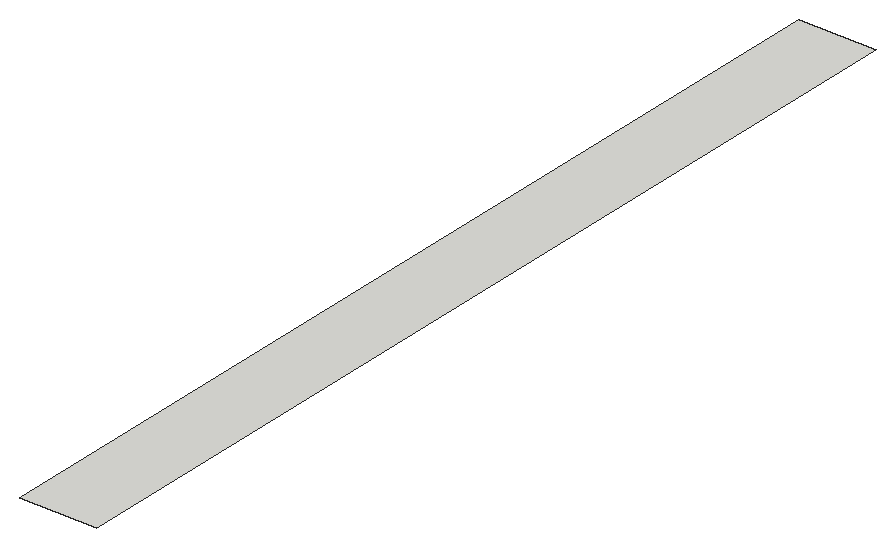
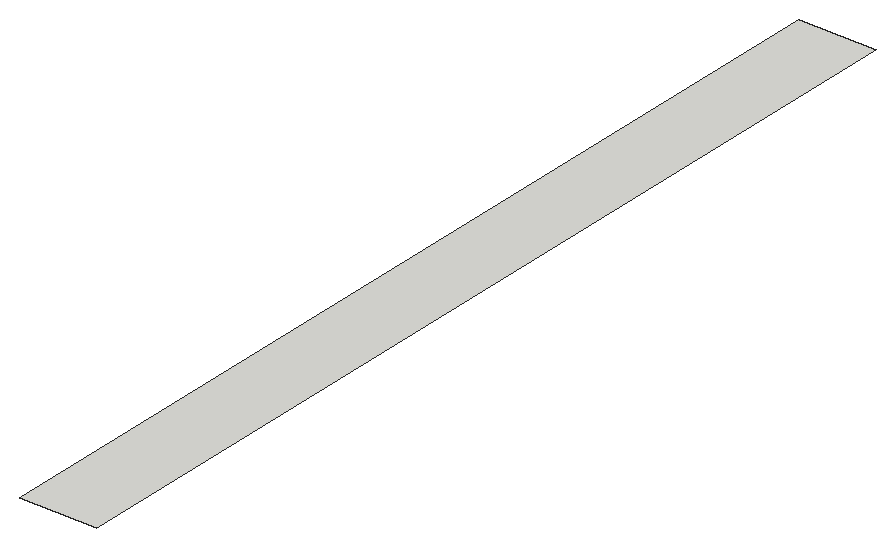
# SketchUp Ruby script. Lengths in inches.
U = 1.inch
M = Sketchup.active_model
def pt(a) = Geom::Point3d.new(a.map { |v| v * U })
def face(e, loops, mat)
  f = e.add_face(loops[0].map { |a| pt(a) })
  loops[1..].each { |l| e.add_face(l.map { |a| pt(a) }).erase! }
  f.material = f.back_material = mat if mat
  f
end
# faces: each face lists its corners as indices into pts; further lists are holes
def faces(e, pts, list, mat = nil) = list.each { |f| face(e, (f[0].is_a?(Array) ? f : [f]).map { |l| l.map { |i| pts[i] } }, mat) }
# xy, xz, yz: faces in a plane at the given z, y or x. An outline is a flat list of corners, or four numbers for a rectangle; further outlines are holes
def ring(l) = l.size == 4 ? [[l[0], l[1]], [l[2], l[1]], [l[2], l[3]], [l[0], l[3]]] : l.each_slice(2).to_a
def flat(e, list, mat, &to3) = list.each { |f| face(e, (f[0].is_a?(Array) ? f : [f]).map { |l| ring(l).map { |u, v| to3.(u, v) } }, mat) }
def xy(e, z, list, mat = nil) = flat(e, list, mat) { |x, y| [x, y, z] }
def xz(e, y, list, mat = nil) = flat(e, list, mat) { |x, z| [x, y, z] }
def yz(e, x, list, mat = nil) = flat(e, list, mat) { |y, z| [x, y, z] }
def lines(e, pts, list) = list.each { |a, b| e.add_line(pt(pts[a]), pt(pts[b])) }
# prism: a flat outline (further loops are holes) pulled along v
def prism(e, loops, v, mat = nil)
  f = face(e, loops, mat); d = Geom::Vector3d.new(v.map { |x| x * U })
  f.pushpull(f.normal.samedirection?(d) ? d.length : -d.length)
end
def box(e, o, s, mat = nil) = prism(e, [[o, [o[0] + s[0], o[1], o[2]], [o[0] + s[0], o[1] + s[1], o[2]], [o[0], o[1] + s[1], o[2]]]], [0, 0, s[2]], mat)
def at(x, y, z, deg = 0) = Geom::Transformation.translation(pt([x, y, z])) * Geom::Transformation.rotation(ORIGIN, Z_AXIS, deg.degrees)
def axes(o, x, y, z) = Geom::Transformation.new([*x, 0, *y, 0, *z, 0, *pt(o).to_a, 1])
def part(name) = M.definitions.add(name)
# library, detail: a bought-in or finely detailed component or shape, given as its bounding box
def library(name, o, s) = part(name).tap { |d| box(d.entities, o, s) }
def detail(e, o, s) = box(e.add_group.entities, o, s)
def put(e, d, t, mat = nil) = e.add_instance(d, t).tap { |i| i.material = mat if mat }
def group(e, t, mat = nil) = e.add_group.tap { |g| g.transformation = t; g.material = mat if mat }.entities
root = M.entities
xy(root,95.625,[[202.72,364.57,211.5,476.15]])
